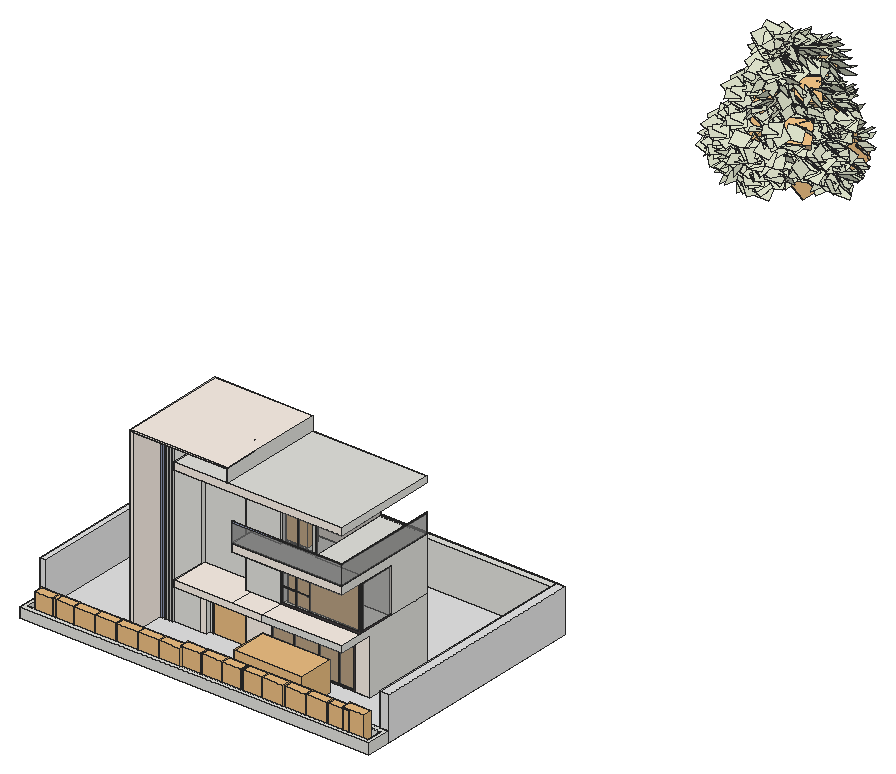
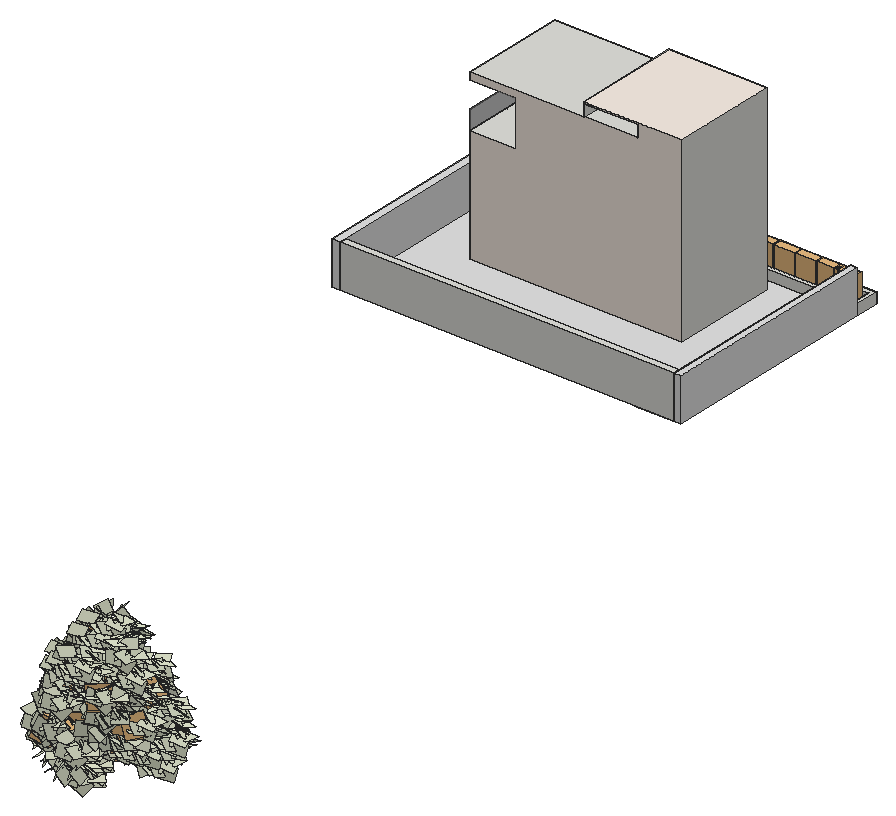
# SketchUp Ruby script. Lengths in inches.
U = 1.inch
M = Sketchup.active_model
def pt(a) = Geom::Point3d.new(a.map { |v| v * U })
def face(e, loops, mat)
  f = e.add_face(loops[0].map { |a| pt(a) })
  loops[1..].each { |l| e.add_face(l.map { |a| pt(a) }).erase! }
  f.material = f.back_material = mat if mat
  f
end
# faces: each face lists its corners as indices into pts; further lists are holes
def faces(e, pts, list, mat = nil) = list.each { |f| face(e, (f[0].is_a?(Array) ? f : [f]).map { |l| l.map { |i| pts[i] } }, mat) }
# xy, xz, yz: faces in a plane at the given z, y or x. An outline is a flat list of corners, or four numbers for a rectangle; further outlines are holes
def ring(l) = l.size == 4 ? [[l[0], l[1]], [l[2], l[1]], [l[2], l[3]], [l[0], l[3]]] : l.each_slice(2).to_a
def flat(e, list, mat, &to3) = list.each { |f| face(e, (f[0].is_a?(Array) ? f : [f]).map { |l| ring(l).map { |u, v| to3.(u, v) } }, mat) }
def xy(e, z, list, mat = nil) = flat(e, list, mat) { |x, y| [x, y, z] }
def xz(e, y, list, mat = nil) = flat(e, list, mat) { |x, z| [x, y, z] }
def yz(e, x, list, mat = nil) = flat(e, list, mat) { |y, z| [x, y, z] }
def lines(e, pts, list) = list.each { |a, b| e.add_line(pt(pts[a]), pt(pts[b])) }
# prism: a flat outline (further loops are holes) pulled along v
def prism(e, loops, v, mat = nil)
  f = face(e, loops, mat); d = Geom::Vector3d.new(v.map { |x| x * U })
  f.pushpull(f.normal.samedirection?(d) ? d.length : -d.length)
end
def box(e, o, s, mat = nil) = prism(e, [[o, [o[0] + s[0], o[1], o[2]], [o[0] + s[0], o[1] + s[1], o[2]], [o[0], o[1] + s[1], o[2]]]], [0, 0, s[2]], mat)
def at(x, y, z, deg = 0) = Geom::Transformation.translation(pt([x, y, z])) * Geom::Transformation.rotation(ORIGIN, Z_AXIS, deg.degrees)
def axes(o, x, y, z) = Geom::Transformation.new([*x, 0, *y, 0, *z, 0, *pt(o).to_a, 1])
def part(name) = M.definitions.add(name)
# library, detail: a bought-in or finely detailed component or shape, given as its bounding box
def library(name, o, s) = part(name).tap { |d| box(d.entities, o, s) }
def detail(e, o, s) = box(e.add_group.entities, o, s)
def put(e, d, t, mat = nil) = e.add_instance(d, t).tap { |i| i.material = mat if mat }
def group(e, t, mat = nil) = e.add_group.tap { |g| g.transformation = t; g.material = mat if mat }.entities
root = M.entities
M.materials.add("Celtis_australis_s cópia1").color = [224, 229, 205]
M.materials.add("Niraj_Shirt").color = [144, 153, 181]
M.materials.add("[0009_Linen]").color = [250, 240, 230]
M.materials.add("[Asphalt New]").color = [67, 60, 62]
M.materials.add("[Polished Concrete Old]").color = [229, 229, 229]
M.materials.add("[Translucent Glass Gray]").color = [128, 128, 128]
M.materials["[Translucent Glass Gray]"].alpha = 0.5
M.materials.add("bark_cherry").color = [99, 76, 62]
c1 = part("leaf1\#1")
p = [[1.6,6.78,0.04],[-9.34,-4.04,0.02],[2.67,-16.2,2.05],[13.62,-5.38,2.07]]
faces(c1.entities,p,[[0,1,2,3]],"Celtis_australis_s cópia1")
c2 = part("leaf_group1\#1")
put(c2.entities,c1,axes([-0.06,3.68,7.3125],[0.53029,-0.80282,-0.27253],[0.82812,0.42159,0.36943],[-0.18168,-0.42159,0.8884]))
put(c2.entities,c1,axes([6.4375,-3.58,5.23],[1,0,0],[0,0.98927,0.14608],[0,-0.14608,0.98927]))
put(c2.entities,c1,axes([-0.99,3.68,1.22],[0.57591,-0.80282,0.15431],[0.36532,0.42159,0.82994],[-0.73135,-0.42159,0.53609]))
put(c2.entities,c1,axes([18.71,8.59,4.39],[0.33053,0.77491,0.53877],[-0.79988,-0.073,0.5957],[0.50094,-0.62785,0.5957]))
put(c2.entities,c1,axes([13.16,0.76,0.89],[0.89618,0.3501,0.27256],[-0.44248,0.65988,0.60727],[0.03275,-0.66482,0.74628]))
put(c2.entities,c1,axes([4.53,7.98,7.3125],[-0.1927,0.94265,-0.27253],[0.88368,0.28746,0.36943],[-0.42658,0.16964,0.8884]))
put(c2.entities,c1,axes([12.46,21.28,7.16],[0.85019,0.38493,0.35918],[0.30538,-0.91629,0.25914],[-0.42887,0.11063,0.89657]))
put(c2.entities,c1,axes([6.53,15.18,2.59],[0.70711,0.70711,0],[0.5,-0.5,0.70711],[-0.5,0.5,0.70711]))
put(c2.entities,c1,axes([-3.17,8.15,3.46],[-0.03719,0.74973,0.66069],[0.94096,-0.19634,0.27576],[-0.33647,-0.63194,0.69817]))
put(c2.entities,c1,axes([23.03,17.79,4.39],[0.78166,-0.31422,0.53877],[-0.61722,-0.51398,0.5957],[-0.08973,0.79818,0.5957]))
put(c2.entities,c1,axes([14.78,21.52,3.21],[0.67246,-0.04394,0.73882],[-0.28657,-0.93583,0.20517],[-0.6824,0.3497,0.64191]))
put(c2.entities,c1,axes([10.37,-1.8125,9],[0.99279,-0.06448,-0.101],[0.11527,0.74421,0.65792],[0.03275,-0.66482,0.74628]))
put(c2.entities,c1,axes([1.45,16.1875,2.9375],[-0.2106,-0.86579,-0.45394],[0.96054,-0.26957,0.06852],[-0.18168,-0.42159,0.8884]))
c3 = library("branch1\#2",[0,0,0],[33.4,33.29,108.01])
c4 = library("plants",[0.18,-0.67,0.63],[15.85,6.49,10.81])
c5 = library("fronceur+aubin+blanc+(3)",[-47.99,-0.29,1.66],[95.37,4.84,114.09])
c6 = library("ประตู",[99.61,0,0],[47.24,8.5625,80.71])
c7 = library("IG4800PR100",[498.85,-116.83,-5.17],[69.93,36.56,30.83])
c8 = part("branch2\#1")
p = [[13.74,0.36,0.5],[11.5,11.3125,10.98],[14.125,0.95,0],[14.97,0.95,0.19],[12.12,10.6875,11.67],[15.1,0.36,0.82],
  [11.05,10.4375,11.49],[14.34,0,1.01],[6.08,18.54,23.51],[6.83,18.32,23.89],[6.09,17.93,24.13],[3.27,29.37,34],
  [3.27,29.68,33.56],[3.73,29.59,33.82],[0,43.16,40.74],[0,43.16,40.75],[0.01,43.16,40.75],[5.59,23.2,32.77],
  [4.65,30.48,39.08],[1.92,39.79,43.02],[5.09,28.47,41.41]]
faces(c8.entities,p,[[0,1,2],[2,1,3],[3,4,5],[3,1,4],[6,0,7],[0,6,1],[5,6,7],[6,5,4],
  [6,8,1],[1,9,4],[9,1,8],[8,6,10],[4,10,6],[10,4,9],[10,11,8],[8,12,9],
  [12,8,11],[10,9,11],[13,11,9],[13,9,12],[14,12,11,15],[12,14,16,13],[13,16,15,11]],"bark_cherry")
lines(c8.entities,p,[[17,18],[11,19],[20,17],[17,10]])
c9 = library("Tenda",[0,0,0],[9.09,66.93,111.26])
c10 = part("branch3")
p = [[6.085,7.082,2.644],[4.083,0.001,0],[4.08,0.002,0.001],[5.841,7.141,2.739],[4.083,0,0.004],[6.032,7.035,2.901],
  [8.234,14.378,3.666],[10.055,21.673,1.937],[8.611,14.241,3.496],[10.247,21.661,2.456],[9.737,21.9,2.346],[9.715,21.803,2.365],
  [12.357,28.999,2.225],[12.894,28.763,2.608],[12.761,28.844,2.204],[10.064,22.087,2.083],[10.362,21.9,2.346],[5.434,16.028,3.111],
  [10.04,22.14,2.516],[12.239,29.014,2.642],[8.553,14.232,3.928],[5.628,15.927,3.273],[5.444,16.098,3.367],[12.571,28.869,2.879],
  [0.628,10.534,6.01],[0.625,10.536,6.008],[0.625,10.537,6.012],[6.135,9.846,4.735],[0.003,10.534,6.01],[0,10.537,6.012],
  [1.761,10.232,4.093],[4.16,5.476,4.049],[3.718,5.459,5.543],[3.205,0.783,1.919]]
faces(c10.entities,p,[[0,1,2,3],[3,2,4,5],[1,0,5,4],[6,7,8],[9,8,7],[7,6,10,11],[12,7,11],[13,7,14],
  [14,7,12],[13,9,7],[15,16,17],[15,17,18],[12,11,19],[20,10,6],[10,20,9,11],[21,17,16],
  [21,16,22],[18,22,16],[9,19,11],[8,9,20],[22,18,17],[9,13,23],[19,9,23],[0,8,5],
  [3,6,0],[8,0,6],[3,5,6],[20,5,8],[20,6,5],[21,24,25,17],[26,22,17,25],[22,26,24,21]],"bark_cherry")
lines(c10.entities,p,[[27,20],[28,29],[17,30],[27,31],[32,27],[5,33]])
c11 = part("branch1\#1")
p = [[23.875,19.65,51.47],[23.47,20.4,51.62],[21.1,21.64,19.5],[21.93,21.1875,19.92],[21.95,22.18,19.69],[26.48,9.62,42.86],
  [30.79,16.22,49.68],[31.01,4.77,55.38],[31.01,0,68.57],[9.91,24.21,59.69],[9.92,24.21,59.7],[24,20.54,51.64],
  [12.85,4.92,53.79],[26.1,8.92,42.74],[31.84,25.13,88.91],[31.84,25.13,106.45],[30.18,33.29,93.95],[30.18,25.42,69.53],
  [0,6.37,81.52],[11.1,10.75,77.87]]
lines(c11.entities,p,[[0,1],[2,3],[3,4],[5,6],[7,8],[9,10],[1,11],[11,0],[12,13],[4,2],[14,15],[16,17],
  [18,19]])
detail(c11.entities,[5.26,2.24,0],[28.14,24.14,108.01])
xy(root,0,[[210.55,62.39,467.66,74.8125],[464.46,77.82,470.67,244.19]])
xy(root,0,[[268.49,86.79,271.14,86.79,271.14,111.79,273.22,111.79,273.22,112.85,274.76,112.85,274.76,111.91,275.98,111.91,275.98,112.85,277.43,112.85,277.43,111.91,278.58,111.91,278.58,112.85,279.57,112.85,279.57,111.91,280.6,111.91,280.6,112.85,305.28,112.85,305.28,116.04,308.52,116.04,308.52,120.22,335.4,120.22,335.4,112.85,428.49,112.85,428.49,167.22,268.49,167.22]],"[0009_Linen]")
xy(root,0,[[212.23,77.82,464.46,238.69],[[268.49,86.79,271.14,86.79,271.14,111.79,273.22,111.79,273.22,112.85,274.76,112.85,274.76,111.91,275.98,111.91,275.98,112.85,277.43,112.85,277.43,111.91,278.58,111.91,278.58,112.85,279.57,112.85,279.57,111.91,280.6,111.91,280.6,112.85,305.28,112.85,305.28,116.04,335.4,116.04,335.4,112.85,428.49,112.85,428.49,167.22,268.49,167.22],[212.23,238.69,241.77,244.19]],[308.52,116.04,335.4,120.22]],"[Polished Concrete Old]")
xy(root,7.6875,[[[207.54,59.38,470.67,77.82],[210.55,62.39,467.66,74.8125]]])
xy(root,32.5,[[212.23,238.69,464.46,244.19]])
xy(root,32.5,[[207.54,77.82,212.23,244.19],[464.46,77.82,470.67,244.19]],"[Polished Concrete Old]")
xy(root,35.8125,[[305.28,112.85,335.4,116.04],[308.52,116.04,335.4,120.22]])
xy(root,41.66,[[301.37,86.79,428.49,112.85]],"[0009_Linen]")
xy(root,46.25,[[368.25,104.41,428.49,104.41,428.49,106.5,426.6875,106.5,426.6875,133.41,368.25,133.41]])
xy(root,46.25,[[301.37,86.79,345.1,86.79,345.1,104.54,341.8,104.54,341.8,115.85,301.62,115.85,301.62,112.85,301.37,112.85],[345.1,86.79,368.25,104.54],[368.25,86.79,428.49,104.41]],"[0009_Linen]")
xy(root,81.17,[[345.1,86.79,368.25,104.54],[368.25,86.79,428.49,104.41],[368.25,104.41,368.25,133.41,426.6875,133.41,426.6875,106.5,428.49,106.5,428.49,104.41]])
xy(root,86.65,[[345.1,87.28,427.89,87.28,427.89,104.54,393.68,104.54,393.68,106.66,368.25,106.66,368.25,104.54,345.1,104.54],[393.68,104.54,427.89,167.22]])
xy(root,87.88,[[369.49,104.54,380.96,106.66],[380.96,104.54,381.57,106.66],[381.57,104.54,392.44,106.66]])
xy(root,101.52,[[345.1,86.79,428.49,86.79,428.49,167.22,427.89,167.22,427.89,87.28,345.1,87.28]])
xy(root,119.85,[[369.49,104.54,380.96,106.66],[380.96,104.54,381.57,106.66],[381.57,104.54,392.44,106.66]])
xy(root,121.24,[[368.25,86.79,428.49,106.66],[393.68,106.66,428.49,167.22]])
xy(root,121.24,[[301.62,86.79,301.62,115.85,341.8,115.85,341.8,104.54,368.25,104.54,368.25,86.79]],"[0009_Linen]")
xy(root,126.27,[[301.62,86.79,341.3,115.85],[342.12,86.79,428.49,167.22],[301.62,115.85,341.3,167.22]])
xy(root,135.71,[[301.62,112.85,341.3,115.85],[301.62,115.85,341.3,167.22]])
xy(root,135.71,[[271.14,86.79,271.14,111.79,273.22,111.79,273.22,112.85,274.76,112.85,274.76,111.91,275.98,111.91,275.98,112.85,277.43,112.85,277.43,111.91,278.58,111.91,278.58,112.85,279.57,112.85,279.57,111.91,280.6,111.91,280.6,112.85,341.3,112.85,341.3,86.79]],"[0009_Linen]")
xy(root,136.77,[[268.49,86.79,342.12,167.22]],"[0009_Linen]")
xz(root,59.38,[[207.54,0,470.67,7.6875]])
xz(root,62.39,[[210.55,0,467.66,7.6875]])
xz(root,74.8125,[[210.55,0,464.46,7.6875],[464.46,0,467.66,7.6875]])
xz(root,77.82,[[212.23,0,464.46,7.6875],[464.46,0,470.67,7.6875]])
xz(root,77.82,[[207.54,7.6875,212.23,32.5],[464.46,7.6875,470.67,32.5]],"[Polished Concrete Old]")
xz(root,86.79,[[368.25,41.66,428.49,46.25],[341.3,126.27,342.12,135.71],[268.49,135.71,271.14,136.77]])
xz(root,86.79,[[345.1,100.56,428.49,101.03,428.49,101.52,345.1,101.52]],"Niraj_Shirt")
xz(root,86.79,[[268.49,0,271.14,135.71],[301.37,41.66,368.25,46.25],[345.1,81.17,428.49,86.26],[301.62,121.24,428.49,126.27],[271.14,135.71,342.12,136.77]],"[0009_Linen]")
xz(root,86.79,[[345.1,86.26,428.49,86.26,428.49,101.03,345.1,100.56]],"[Translucent Glass Gray]")
xz(root,87.28,[[345.1,86.65,427.89,101.52]],"[Translucent Glass Gray]")
xz(root,104.41,[[[368.25,46.25,428.49,81.17],[369.53,47.53,427.21,79.89]],[379.66,47.53,380.15,58.18],[389.78,47.53,390.375,79.89],[369.53,58.18,379.66,58.7],[379.66,58.18,380.15,58.7],
  [380.15,58.18,389.78,58.7],[379.66,58.7,380.15,73.27],[369.53,73.27,379.66,73.75],[379.66,73.27,380.15,73.75],[380.15,73.27,389.78,73.75],
  [379.66,73.75,380.15,79.89]],"[Asphalt New]")
xz(root,104.41,[[369.53,47.53,379.66,58.18],[380.15,47.53,389.78,58.18],[390.375,47.53,427.21,79.89],[369.53,58.7,379.66,73.27],[380.15,58.7,389.78,73.27],
  [369.53,73.75,379.66,79.89],[380.15,73.75,389.78,79.89]],"[Translucent Glass Gray]")
xz(root,104.54,[[341.8,46.25,368.25,46.25,368.25,81.17,345.1,81.17,345.1,86.65,368.25,86.65,368.25,121.24,341.8,121.24],[380.96,87.88,381.57,119.85]])
xz(root,104.54,[[369.49,87.88,380.96,119.85],[381.57,87.88,392.44,119.85]],"[Translucent Glass Gray]")
xz(root,106.5,[[426.6875,46.25,428.49,81.17]],"[Translucent Glass Gray]")
xz(root,106.66,[[[368.25,86.65,393.68,121.24],[369.49,87.88,392.44,119.85]]],"[Asphalt New]")
xz(root,111.79,[[271.14,0,273.22,135.71]],"Niraj_Shirt")
xz(root,111.91,[[274.76,0,275.98,135.71],[277.43,0,278.58,135.71],[279.57,0,280.6,135.71]],"[Asphalt New]")
xz(root,112.85,[[273.22,0,274.76,135.71],[275.98,0,277.43,135.71],[278.58,0,279.57,135.71],[280.6,0,301.37,0,301.37,46.25,301.62,46.25,301.62,135.71,280.6,135.71]])
xz(root,112.85,[[301.37,0,305.28,0,305.28,35.8125,335.4,35.8125,335.4,0,353.91,0,353.91,39.8,418.03,39.8,418.03,0,428.49,0,428.49,41.66,301.37,41.66]],"[0009_Linen]")
xz(root,112.85,[[353.91,0,381.1,0,381.1,1.17,355.08,1.17,355.08,38.625,416.86,38.625,416.86,1.17,381.1,1.17,381.1,0,418.03,0,418.03,39.8,353.91,39.8],[371.29,1.17,371.83,30.06],[390.36,1.17,390.91,30.06],[405.25,1.17,405.7,30.06],[355.08,30.06,371.29,30.59],
  [371.29,30.06,371.83,30.59],[371.83,30.06,390.36,30.59],[390.36,30.06,390.91,30.59],[390.91,30.06,405.25,30.59],[405.25,30.06,405.7,30.59],
  [405.7,30.06,416.86,30.59],[371.29,30.59,371.83,38.625],[390.36,30.59,390.91,38.625],[405.25,30.59,405.7,38.625]],"[Asphalt New]")
xz(root,112.85,[[355.08,1.17,371.29,30.06],[371.83,1.17,390.36,30.06],[390.91,1.17,405.25,30.06],[405.7,1.17,416.86,30.06],[355.08,30.59,371.29,38.625],
  [371.83,30.59,390.36,38.625],[390.91,30.59,405.25,38.625],[405.7,30.59,416.86,38.625]],"[Translucent Glass Gray]")
xz(root,115.85,[[301.62,46.25,332.27,121.24],[301.62,121.24,332.27,126.27],[332.27,121.24,341.8,121.24,341.8,135.71,341.3,135.71,341.3,126.27,332.27,126.27],[301.62,126.27,332.27,135.71]])
xz(root,115.85,[[332.27,46.25,341.8,46.25,341.8,121.24,332.27,121.24,332.27,101.26,333.23,101.26,333.23,120.28,340.84,120.28,340.84,47.21,333.23,47.21,333.23,100.65,332.27,100.65],[333.23,77.05,340.84,77.8],[332.27,100.65,333.23,101.26],[333.23,100.65,340.84,101.26],[[332.27,126.27,341.3,135.71],[332.79,126.8,340.77,135.1875]]],"[Asphalt New]")
xz(root,115.85,[[333.23,47.21,340.84,77.05],[333.23,77.8,340.84,100.65],[333.23,101.26,340.84,120.28],[332.79,126.8,340.77,135.1875]],"[Translucent Glass Gray]")
xz(root,116.04,[[305.28,0,308.52,35.8125]])
xz(root,120.22,[[308.52,0,335.4,35.8125]])
xz(root,133.41,[[368.25,46.25,426.6875,81.17]])
xz(root,167.22,[[427.89,86.65,428.49,101.52]])
xz(root,167.22,[[[268.49,0,268.49,136.77,342.12,136.77,342.12,126.27,428.49,126.27,428.49,121.24,393.68,121.24,393.68,86.65,428.49,86.65,428.49,0],[301.62,126.27,341.3,135.71]]],"[0009_Linen]")
xz(root,238.69,[[212.23,0,464.46,32.5]])
xz(root,244.19,[[212.23,0,464.46,32.5]])
xz(root,244.19,[[207.54,0,212.23,32.5],[464.46,0,470.67,32.5]],"[Polished Concrete Old]")
yz(root,207.54,[[59.38,0,77.82,7.6875]])
yz(root,207.54,[[77.82,0,244.19,32.5]],"[Polished Concrete Old]")
yz(root,210.55,[[62.39,0,74.8125,7.6875]])
yz(root,212.23,[[238.69,0,244.19,32.5]])
yz(root,212.23,[[77.82,0,238.69,32.5]],"[Polished Concrete Old]")
yz(root,268.49,[[86.79,0,167.22,136.77]])
yz(root,271.14,[[86.79,0,111.79,135.71]],"[0009_Linen]")
yz(root,273.22,[[111.79,0,112.85,135.71]],"Niraj_Shirt")
yz(root,274.76,[[111.91,0,112.85,135.71]])
yz(root,275.98,[[111.91,0,112.85,135.71]])
yz(root,277.43,[[111.91,0,112.85,135.71]])
yz(root,278.58,[[111.91,0,112.85,135.71]])
yz(root,279.57,[[111.91,0,112.85,135.71]])
yz(root,280.6,[[111.91,0,112.85,135.71]])
yz(root,301.37,[[86.79,41.66,112.85,46.25]])
yz(root,301.62,[[112.85,46.25,115.85,121.24],[86.79,121.24,112.85,126.27],[112.85,121.24,115.85,126.27],[112.85,126.27,115.85,135.71],[115.85,126.27,167.22,135.71]])
yz(root,305.28,[[112.85,0,116.04,35.8125]])
yz(root,308.52,[[116.04,0,120.22,35.8125]])
yz(root,335.4,[[112.85,0,116.04,35.8125],[116.04,0,120.22,35.8125]])
yz(root,341.3,[[86.79,126.27,115.85,135.71],[115.85,126.27,167.22,135.71]])
yz(root,341.8,[[104.54,46.25,115.85,117.92],[104.54,117.92,115.85,121.24]])
yz(root,342.12,[[86.79,126.27,167.22,126.27,167.22,136.77,112.85,136.77,112.85,135.71,86.79,135.71],[86.79,135.71,112.85,136.77]])
yz(root,345.1,[[86.79,81.17,86.79,101.52,87.28,101.52,87.28,86.65,104.54,86.65,104.54,81.17]])
yz(root,368.25,[[104.41,46.25,104.54,81.17],[104.54,46.25,133.41,81.17],[104.54,86.65,106.66,121.24]])
yz(root,369.49,[[104.54,87.88,106.66,119.85]])
yz(root,392.44,[[104.54,87.88,106.66,119.85]])
yz(root,393.68,[[106.66,86.65,167.22,121.24]],"[Translucent Glass Gray]")
yz(root,427.89,[[87.28,86.65,167.22,101.52]],"[Translucent Glass Gray]")
yz(root,428.49,[[112.85,0,167.22,0,167.22,46.25,86.79,46.25,86.79,41.66,112.85,41.66],[133.41,46.25,167.22,46.25,167.22,86.26,86.79,86.26,86.79,81.17,133.41,81.17],[86.79,121.24,167.22,126.27]])
yz(root,428.49,[[167.22,100.56,167.22,101.52,86.79,101.52,86.79,101.03]],"Niraj_Shirt")
yz(root,428.49,[[104.41,46.25,105.46,47.8125],[105.46,46.25,106.5,47.8125],[106.5,46.25,133.41,47.8125],[104.41,47.8125,105.46,79.97],[105.46,47.8125,106.5,79.97],
  [104.41,79.97,105.46,81.17],[105.46,79.97,106.5,81.17],[106.5,79.97,133.41,81.17]],"[Asphalt New]")
yz(root,428.49,[[106.5,47.8125,133.41,79.97],[86.79,86.26,167.22,86.26,167.22,100.56,86.79,101.03]],"[Translucent Glass Gray]")
yz(root,464.46,[[77.82,0,238.69,32.5],[238.69,0,244.19,32.5]],"[Polished Concrete Old]")
yz(root,467.66,[[62.39,0,74.8125,7.6875]])
yz(root,470.67,[[59.38,0,77.82,7.6875]])
yz(root,470.67,[[77.82,0,244.19,32.5]],"[Polished Concrete Old]")
p = [[426.6875,106.5,81.17],[426.6875,106.5,86.65],[426.6875,133.41,81.17],[426.6875,133.41,86.65],[341.8,104.54,121.24],[341.8,104.54,126.27],
  [230.87,755.93,87.79],[230.87,758.68,81.77],[230.08,749.41,85.86],[230.08,750.25,86.8],[230.55,755.93,83.6],[230.55,752.92,83.6],
  [230.55,751.66,81.77],[230.08,751.96,86.8]]
lines(root,p,[[0,1],[2,3],[4,5],[6,7],[8,9],[10,11],[12,11],[13,9]])
put(root,c2,axes([216.06,797.23,-3.38],[-0.02633,-0.60304,-0.08806],[0.60942,-0.02661,0],[-0.00384,-0.08797,0.60361]))
put(root,c2,axes([226.28,784.04,-3.38],[-0.02633,-0.60304,-0.08806],[0.60942,-0.02661,0],[-0.00384,-0.08797,0.60361]))
put(root,c3,axes([238.02,760.1,-14.24],[-0.33685,0.35002,0.0465],[-0.16871,-0.216,0.40376],[0.27917,0.23636,0.24309]))
put(root,c2,axes([188.76,752.55,-4.8],[0.3991,-0.46073,-0.02342],[0.46107,0.39939,0],[0.01533,-0.0177,0.60955]))
put(root,c2,axes([254.06,777.32,1.42],[-0.03264,0.60273,-0.08806],[-0.60911,-0.03299,0],[-0.00476,0.08793,0.60361]))
put(root,c2,axes([247.84,777.32,1.42],[-0.03264,0.60273,-0.08806],[-0.60911,-0.03299,0],[-0.00476,0.08793,0.60361]))
put(root,c2,axes([266.26,762.1,3.33],[-0.40779,0.44503,-0.08806],[-0.44974,-0.41211,0],[-0.05949,0.06492,0.60361]))
put(root,c2,axes([216.06,790.03,3.48],[-0.02633,-0.60304,-0.08806],[0.60942,-0.02661,0],[-0.00384,-0.08797,0.60361]))
put(root,c2,axes([233.16,790.72,4.77],[0.02633,0.60304,-0.08806],[-0.60942,0.02661,0],[0.00384,0.08797,0.60361]))
put(root,c2,axes([232.93,728.81,6.38],[-0.28191,0.53555,0.07626],[-0.54094,-0.27848,-0.04403],[-0.00384,-0.08797,0.60361]))
put(root,c3,axes([223.71,776.8,-3.29],[-0.1895,-0.44786,-0.04063],[0.30296,-0.15972,0.34763],[-0.29911,0.0988,0.30606]))
put(root,c2,axes([249.16,762.41,7.6],[0.40779,-0.44503,-0.08806],[0.44974,0.41211,0],[0.05949,-0.06492,0.60361]))
put(root,c2,axes([227.4375,746.57,8.31],[0.60361,0,-0.08806],[0,0.61,0],[0.08806,0,0.60361]))
put(root,c2,axes([189.59,739.46,8.77],[0.40732,0.44546,-0.08806],[-0.45017,0.41163,0],[0.05942,0.06499,0.60361]))
put(root,c2,axes([222.45,790.72,9.01],[0.02633,0.60304,-0.08806],[-0.60942,0.02661,0],[0.00384,0.08797,0.60361]))
put(root,c2,axes([250.11,787.02,9.04],[-0.02633,-0.60304,-0.08806],[0.60942,-0.02661,0],[-0.00384,-0.08797,0.60361]))
put(root,c2,axes([192.04,762.54,7.13],[0.3991,-0.46073,-0.02342],[0.46107,0.39939,0],[0.01533,-0.0177,0.60955]))
put(root,c2,axes([206.43,772.22,10.21],[0.36326,-0.48206,-0.08806],[0.48717,0.36711,0],[0.05299,-0.07033,0.60361]))
put(root,c2,axes([245.47,792.01,16.88],[0.0268,-0.60304,-0.08792],[0.5076,-0.02661,0.33725],[-0.33723,-0.08797,0.50063]))
put(root,c2,axes([236.02,723.42,15.2],[0.18169,0.56367,-0.14615],[-0.57554,0.19712,0.04474],[0.08857,0.12457,0.59054]))
put(root,c2,axes([212.23,728.7,15.2],[0.36326,-0.46774,-0.14615],[0.48717,0.36437,0.04474],[0.05299,-0.14336,0.59054]))
put(root,c2,axes([257.07,772.21,11.98],[-0.03264,0.60273,-0.08806],[-0.60911,-0.03299,0],[-0.00476,0.08793,0.60361]))
put(root,c4,axes([309.81,63.04,-1.2],[1,0,0],[0,1,0],[0,0,1.81]))
put(root,c4,axes([293.68,63.04,-1.2],[1,0,0],[0,1,0],[0,0,1.81]))
put(root,c4,axes([277.56,63.04,-1.2],[1,0,0],[0,1,0],[0,0,1.81]))
put(root,c4,axes([261.43,63.04,-1.2],[1,0,0],[0,1,0],[0,0,1.81]))
put(root,c4,axes([245.31,63.04,-1.2],[1,0,0],[0,1,0],[0,0,1.81]))
put(root,c4,axes([229.18,63.04,-1.2],[1,0,0],[0,1,0],[0,0,1.81]))
put(root,c4,axes([215.93,63.04,-1.2],[1,0,0],[0,1,0],[0,0,1.81]))
put(root,c5,axes([385.02,115.68,-0.58],[0.67202,0,0],[0,0.28,0],[0,0,0.34887]))
put(root,c6,axes([250.52,116.04,0],[0.576,0,0],[0,0.23357,0],[0,0,0.4416]))
put(root,c7,axes([-8.66,161.63,3.77],[0.73,0,0],[0,0.73,0],[0,0,0.73]))
put(root,c2,axes([195.81,772.24,12.16],[0.36326,-0.48206,-0.08806],[0.48717,0.36711,0],[0.05299,-0.07033,0.60361]))
put(root,c2,axes([213.6875,770.92,17.05],[0.5135,0.31129,0.1073],[-0.28515,0.51982,-0.14344],[-0.16464,0.07059,0.58311]))
put(root,c4,axes([403.72,64.4,0.07],[1,0,0],[0,1,0],[0,0,1.81]))
put(root,c4,axes([419.16,64.4,0.07],[1,0,0],[0,1,0],[0,0,1.81]))
put(root,c4,axes([436.29,64.4,0.07],[1,0,0],[0,1,0],[0,0,1.81]))
put(root,c4,axes([370.41,64.4,0.07],[1,0,0],[0,1,0],[0,0,1.81]))
put(root,c4,axes([356.29,64.4,0.07],[1,0,0],[0,1,0],[0,0,1.81]))
put(root,c4,axes([340.22,64.4,0.07],[1,0,0],[0,1,0],[0,0,1.81]))
put(root,c4,axes([325.1,64.4,0.07],[1,0,0],[0,1,0],[0,0,1.81]))
put(root,c4,axes([386.47,64.4,0.07],[1,0,0],[0,1,0],[0,0,1.81]))
put(root,c2,axes([227.4375,722.97,13.53],[0.60361,0,-0.08806],[0,0.61,0],[0.08806,0,0.60361]))
put(root,c4,axes([447.51,64.4,1.78],[1,0,0],[0,1,0],[0,0,1.81]))
put(root,c2,axes([179.89,752.88,15.29],[0.37986,-0.46909,-0.08806],[0.47406,0.38389,0],[0.05542,-0.06843,0.60361]))
put(root,c2,axes([190.38,736.19,15.29],[0.60361,0,-0.08806],[0,0.61,0],[0.08806,0,0.60361]))
put(root,c2,axes([212.23,727.09,19.95],[0.36326,-0.47815,0.1073],[0.48717,0.33792,-0.14344],[0.05299,0.17111,0.58311]))
put(root,c2,axes([216.06,803.03,16.52],[-0.02633,-0.60304,-0.08806],[0.60942,-0.02661,0],[-0.00384,-0.08797,0.60361]))
put(root,c3,axes([233.28,752.12,5.87],[-0.45329,0.17613,0.04063],[0.15066,0.30756,0.34763],[-0.0746,-0.25058,0.25403]))
put(root,c2,axes([257.07,750.51,18.69],[-0.03264,0.60273,-0.08806],[-0.60911,-0.03299,0],[-0.00476,0.08793,0.60361]))
put(root,c2,axes([249.03,740.77,18.69],[0.51955,0.30726,-0.08806],[-0.31052,0.52505,0],[0.07579,0.04482,0.60361]))
put(root,c2,axes([250.11,792.01,19.375],[-0.02633,-0.60304,-0.08806],[0.60942,-0.02661,0],[-0.00384,-0.08797,0.60361]))
put(root,c2,axes([190.38,739.43,20.28],[0.60361,0,-0.08806],[0,0.61,0],[0.08806,0,0.60361]))
put(root,c2,axes([200.55,764.61,21.35],[0.51021,0.32254,-0.08806],[-0.32595,0.51561,0],[0.07443,0.04705,0.60361]))
put(root,c2,axes([212.23,742.81,25.34],[0.36326,-0.46774,-0.14615],[0.48717,0.36437,0.04474],[0.05299,-0.14336,0.59054]))
put(root,c2,axes([226.99,714.38,26.09],[0.5135,0.31129,0.1073],[-0.28515,0.51982,-0.14344],[-0.16464,0.07059,0.58311]))
put(root,c3,axes([240.04,763.26,10.18],[-0.39301,-0.28642,0.04063],[-0.17751,0.29289,0.34763],[0.17063,-0.1981,0.25403]))
put(root,c2,axes([213.6875,770.92,26.47],[0.5135,0.31129,0.1073],[-0.28515,0.51982,-0.14344],[-0.16464,0.07059,0.58311]))
put(root,c2,axes([202.57,763.65,43.84],[0.22637,-0.48206,-0.29744],[0.37806,0.36711,-0.30724],[0.42181,-0.07033,0.43501]))
put(root,c2,axes([191.9375,764.61,24.78],[0.51021,0.32254,-0.08806],[-0.32595,0.51561,0],[0.07443,0.04705,0.60361]))
put(root,c2,axes([244.85,752.02,24.87],[-0.02633,-0.60304,-0.08806],[0.60942,-0.02661,0],[-0.00384,-0.08797,0.60361]))
put(root,c2,axes([212.23,741.19,30.09],[0.36326,-0.47815,0.1073],[0.48717,0.33792,-0.14344],[0.05299,0.17111,0.58311]))
put(root,c2,axes([261.94,752.71,26.16],[0.02633,0.60304,-0.08806],[-0.60942,0.02661,0],[0.00384,0.08797,0.60361]))
put(root,c3,axes([219.75,753.54,14.49],[-0.08416,0.47897,0.04063],[0.34113,0.03045,0.34763],[-0.25298,-0.066,0.25403]))
put(root,c2,axes([227.4375,722.97,27.22],[0.60361,0,-0.08806],[0,0.61,0],[0.08806,0,0.60361]))
put(root,c2,axes([190.38,736.19,27.22],[0.60361,0,-0.08806],[0,0.61,0],[0.08806,0,0.60361]))
put(root,c2,axes([228.02,761.94,30.28],[-0.02633,-0.60304,-0.08806],[0.60942,-0.02661,0],[-0.00384,-0.08797,0.60361]))
put(root,c2,axes([250.07,765.02,30.43],[-0.02633,-0.60304,-0.08806],[0.60942,-0.02661,0],[-0.00384,-0.08797,0.60361]))
put(root,c2,axes([217.43,738.3,30.85],[0.36326,-0.48206,-0.08806],[0.48717,0.36711,0],[0.05299,-0.07033,0.60361]))
put(root,c3,axes([229.41,778.87,18.83],[0.22547,-0.43088,0.04063],[-0.31582,-0.13249,0.34763],[0.17242,0.10891,0.19814]))
put(root,c2,axes([188.06,772.22,31.375],[0.36326,-0.48206,-0.08806],[0.48717,0.36711,0],[0.05299,-0.07033,0.60361]))
put(root,c2,axes([249.09,759.85,31.625],[0.02633,0.60304,-0.08806],[-0.60942,0.02661,0],[0.00384,0.08797,0.60361]))
put(root,c2,axes([256.25,774.59,31.84],[-0.51021,0.32254,-0.08806],[-0.32595,-0.51561,0],[-0.07443,0.04705,0.60361]))
put(root,c2,axes([199.8,763.65,32.73],[0.36342,-0.48206,-0.08742],[0.48717,0.36711,0.00085],[0.05194,-0.07033,0.6037]))
put(root,c2,axes([239.14,723.13,33.33],[-0.28191,0.53555,0.07626],[-0.54094,-0.27848,-0.04403],[-0.00384,-0.08797,0.60361]))
put(root,c2,axes([208.43,785.8,35.7],[-0.02987,-0.598,0.11665],[0.58097,0.00722,0.1858],[-0.18352,0.1202,0.56919]))
put(root,c2,axes([242.13,733.78,34.55],[0.36451,0.48112,-0.08806],[-0.48621,0.36837,0],[0.05318,0.07019,0.60361]))
put(root,c2,axes([211.53,776.16,35.65],[0.0258,0.60441,0.07827],[-0.59056,0.00543,0.15267],[0.15058,-0.08224,0.58538]))
put(root,c2,axes([226.99,735.31,39.24],[0.5135,0.31129,0.1073],[-0.28515,0.51982,-0.14344],[-0.16464,0.07059,0.58311]))
put(root,c3,axes([228.08,779.625,24.5],[-0.3624,-0.31691,0.02144],[0.21915,-0.22592,0.36491],[-0.17704,0.21881,0.2418]))
put(root,c2,axes([204.21,793.57,58.73],[0.22637,-0.48206,-0.29744],[0.37806,0.36711,-0.30724],[0.42181,-0.07033,0.43501]))
put(root,c2,axes([251.59,769.62,39.2],[0.36451,0.48112,-0.08806],[-0.48621,0.36837,0],[0.05318,0.07019,0.60361]))
put(root,c2,axes([201.65,793.16,41.875],[-0.02987,-0.598,0.11665],[0.58097,0.00722,0.1858],[-0.18352,0.1202,0.56919]))
put(root,c2,axes([194.92,753.73,40.71],[0.60361,0,-0.08806],[0,0.61,0],[0.08806,0,0.60361]))
put(root,c2,axes([214.32,752.14,40.71],[-0.60361,0,-0.08806],[0,-0.61,0],[-0.08806,0,0.60361]))
put(root,c2,axes([232.95,795.6,40.84],[-0.02633,-0.60304,-0.08806],[0.60942,-0.02661,0],[-0.00384,-0.08797,0.60361]))
put(root,c2,axes([227.74,776.2,40.35],[-0.28191,0.53555,0.07626],[-0.54094,-0.27848,-0.04403],[-0.00384,-0.08797,0.60361]))
put(root,c2,axes([205.82,733.21,41.58],[0.60355,0.00843,-0.08806],[-0.00852,0.60994,0],[0.08805,0.00123,0.60361]))
put(root,c3,axes([231.36,756.4375,29.59],[-0.45329,0.17613,0.04063],[0.15066,0.30756,0.34763],[-0.05819,-0.19545,0.19814]))
put(root,c2,axes([233.41,777.18,43.88],[0.59201,-0.11778,-0.08806],[0.11903,0.59828,0],[0.08636,-0.01718,0.60361]))
put(root,c2,axes([233.41,735.89,43.88],[0.59201,-0.11778,-0.08806],[0.11903,0.59828,0],[0.08636,-0.01718,0.60361]))
put(root,c2,axes([218.57,738.39,49.38],[0.59804,-0.05416,0.1073],[0.07896,0.58761,-0.14344],[-0.09063,0.15452,0.58311]))
put(root,c2,axes([240.9,783.97,46.36],[-0.02633,-0.60304,-0.08806],[0.60942,-0.02661,0],[-0.00384,-0.08797,0.60361]))
put(root,c2,axes([194.92,758.73,47.27],[0.60361,0,-0.08806],[0,0.61,0],[0.08806,0,0.60361]))
put(root,c2,axes([239.23,762.49,47.32],[0.36451,0.48112,-0.08806],[-0.48621,0.36837,0],[0.05318,0.07019,0.60361]))
put(root,c3,axes([226.23,781.73,46.83],[-0.31439,-0.37101,0.04063],[0.24157,-0.24277,-0.34763],[0.16577,-0.11878,0.19814]))
put(root,c2,axes([240.19,771.02,47.39],[-0.28731,-0.53084,-0.08806],[0.53646,-0.29036,0],[-0.04191,-0.07744,0.60361]))
put(root,c2,axes([214.06,784.43,47.75],[-0.28191,0.53555,0.07626],[-0.54094,-0.27848,-0.04403],[-0.00384,-0.08797,0.60361]))
put(root,c2,axes([214.06,776.2,47.75],[-0.28191,0.53555,0.07626],[-0.54094,-0.27848,-0.04403],[-0.00384,-0.08797,0.60361]))
put(root,c2,axes([210.85,745.96,48.8],[0.36326,-0.48206,-0.08806],[0.48717,0.36711,0],[0.05299,-0.07033,0.60361]))
put(root,c2,axes([233.22,758.64,54.63],[0.36326,-0.48206,-0.08806],[-0.48717,-0.36711,0],[0.05299,-0.07033,0.60361]))
put(root,c2,axes([235.36,758.64,54.63],[0.36326,-0.48206,-0.08806],[-0.48717,-0.36711,0],[0.05299,-0.07033,0.60361]))
put(root,c2,axes([201.5,740.7,54.97],[0.59201,-0.11778,-0.08806],[0.11903,0.59828,0],[0.08636,-0.01718,0.60361]))
put(root,c2,axes([200.22,794.83,55.77],[-0.02633,-0.60304,-0.08806],[0.60942,-0.02661,0],[-0.00384,-0.08797,0.60361]))
put(root,c2,axes([199.8,767.95,57.02],[0.36342,-0.48206,-0.08742],[0.48717,0.36711,0.00085],[0.05194,-0.07033,0.6037]))
put(root,c2,axes([230.79,773.98,57.83],[0.36326,-0.48206,-0.08806],[0.48717,0.36711,0],[0.05299,-0.07033,0.60361]))
put(root,c3,axes([222.97,776.375,45.89],[0.29812,-0.21846,0.03088],[-0.1711,-0.19615,0.2642],[0.10389,0.16901,0.19275]))
put(root,c2,axes([209.05,750.375,58.0625],[0.57073,-0.19652,-0.08806],[0.1986,0.57677,0],[0.08326,-0.02867,0.60361]))
put(root,c8,axes([222.81,773.16,55.04],[0.18126,-0.43332,0],[-0.3911,-0.1636,-0.20221],[-0.13245,-0.0554,0.301]))
put(root,c2,axes([220.23,783.01,58.82],[0.36326,-0.48206,-0.08806],[0.48717,0.36711,0],[0.05299,-0.07033,0.60361]))
put(root,c9,axes([333.3,123.68,47.21],[-0.07908,-0.49371,0],[0.10862,-0.0174,0],[0,0,0.80046]))
put(root,c5,axes([400.33,104.74,48.33],[0.56722,0,0],[0,0.28,0],[0,0,0.28]))
put(root,c2,axes([222.9,767.88,60.92],[0.36326,-0.48206,-0.08806],[0.48717,0.36711,0],[0.05299,-0.07033,0.60361]))
put(root,c2,axes([230.79,761.89,60.92],[0.36326,-0.48206,-0.08806],[0.48717,0.36711,0],[0.05299,-0.07033,0.60361]))
put(root,c2,axes([233.22,758.64,60.92],[0.36326,-0.48206,-0.08806],[-0.48717,-0.36711,0],[0.05299,-0.07033,0.60361]))
put(root,c2,axes([227.1,788.2,61.26],[0.36326,-0.48206,-0.08806],[0.48717,0.36711,0],[0.05299,-0.07033,0.60361]))
put(root,c2,axes([205.51,767.95,82.69],[0.22637,-0.48206,-0.29744],[0.37806,0.36711,-0.30724],[0.42181,-0.07033,0.43501]))
put(root,c8,axes([218.69,765.38,61.94],[0.45653,0.11045,0],[0.09969,-0.41206,-0.20221],[0.04755,-0.19654,0.42394]))
put(root,c2,axes([220.23,791.48,68.2],[0.36326,-0.48206,-0.08806],[0.48717,0.36711,0],[0.05299,-0.07033,0.60361]))
put(root,c2,axes([227.32,783.01,69.12],[0.36326,-0.48206,-0.08806],[0.48717,0.36711,0],[0.05299,-0.07033,0.60361]))
put(root,c2,axes([217.1875,747.75,69.29],[0.36342,-0.48206,-0.08742],[0.48717,0.36711,0.00085],[0.05194,-0.07033,0.6037]))
put(root,c2,axes([204.62,771.49,71.58],[0.11324,-0.59299,-0.08742],[0.59919,0.1143,0.00085],[0.01555,-0.08603,0.6037]))
put(root,c2,axes([220.51,741.9,73.37],[0.54973,0.2495,-0.08742],[-0.25199,0.55552,0.00085],[0.07996,0.03535,0.6037]))
put(root,c2,axes([220.42,779.06,74],[0.57905,-0.17042,-0.08806],[0.17223,0.58518,0],[0.08447,-0.02486,0.60361]))
put(root,c8,axes([223.48,772.51,64.07],[0.13597,-0.43332,-0.11987],[-0.4271,-0.1636,0.10696],[0.0997,-0.0554,0.31337]))
put(root,c2,axes([227.51,756.32,76.04],[0.6013,0.05379,-0.08742],[-0.05423,0.60758,0.00085],[0.08715,0.00693,0.6037]))
put(root,c8,axes([231.26,764.95,68.49],[-0.36554,-0.01429,-0.14779],[-0.02221,0.24277,0.03146],[-0.12108,-0.05052,0.30435]))
put(root,c2,axes([219.97,772.03,79.18],[0.36326,-0.48206,-0.08806],[0.48717,0.36711,0],[0.05299,-0.07033,0.60361]))
put(root,c8,axes([223.57,761.81,71.04],[0.24149,0.16992,-0.01936],[0.09506,-0.14279,-0.06752],[0.06488,-0.06591,0.23072]))
put(root,c10,axes([239.26,762.32,73.07],[-0.1028,0.41224,-0.04263],[-0.3808,-0.11129,-0.1579],[-0.16355,0,0.39444]))
put(root,c2,axes([226.39,759.92,78.56],[-0.17143,-0.58182,0.06474],[0.58488,-0.16735,0.04484],[-0.02501,0.07467,0.6049]))
put(root,c2,axes([219.97,762.2,83.68],[0.36326,-0.48206,-0.08806],[0.48717,0.36711,0],[0.05299,-0.07033,0.60361]))
put(root,c11,axes([232.36,764.34,71.86],[-0.12001,0.08573,0.02322],[-0.06888,-0.11448,0.06665],[0.04182,0.03197,0.09812]))
put(root,c10,axes([220.67,745.61,73.5],[0.61,0,0],[0,0.61,0],[0,0,0.61]))
put(root,c10,axes([229.5,764.21,89.76],[-0.44291,-0.09719,-0.14413],[0.13683,0.04845,-0.45312],[0.10723,-0.46324,-0.01716]))
put(root,c9,axes([365.98,121.29,85.68],[0,-1,0],[0.24885,0,0],[0,0,0.32]))
